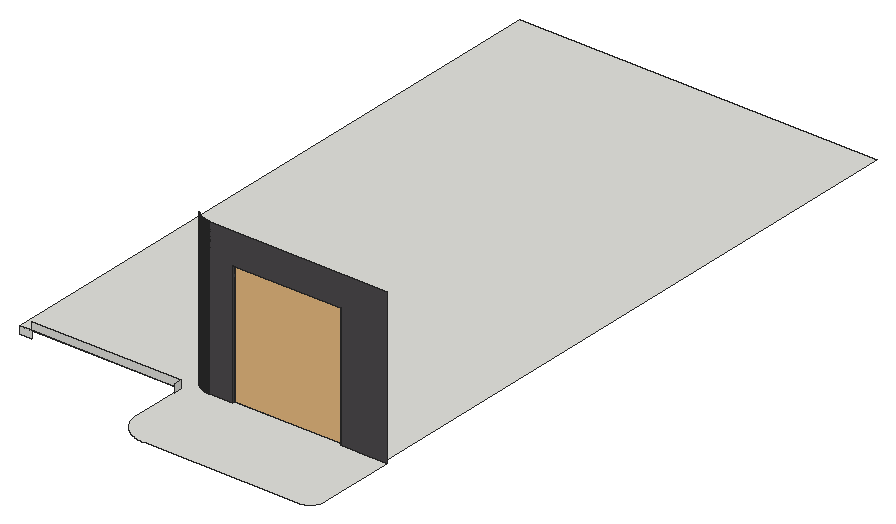
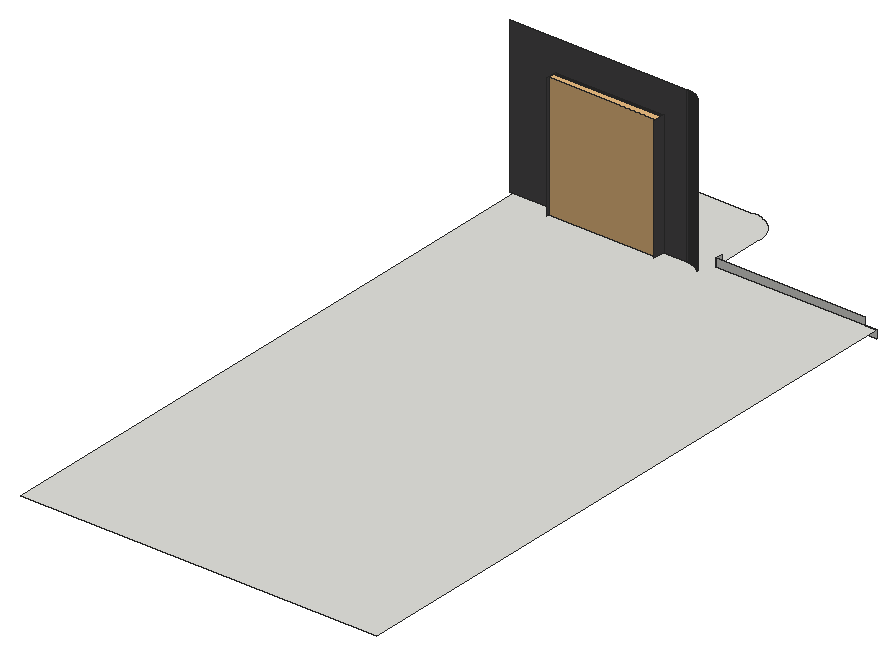
# SketchUp Ruby script. Lengths in inches.
U = 1.inch
M = Sketchup.active_model
def pt(a) = Geom::Point3d.new(a.map { |v| v * U })
def face(e, loops, mat)
  f = e.add_face(loops[0].map { |a| pt(a) })
  loops[1..].each { |l| e.add_face(l.map { |a| pt(a) }).erase! }
  f.material = f.back_material = mat if mat
  f
end
# faces: each face lists its corners as indices into pts; further lists are holes
def faces(e, pts, list, mat = nil) = list.each { |f| face(e, (f[0].is_a?(Array) ? f : [f]).map { |l| l.map { |i| pts[i] } }, mat) }
# xy, xz, yz: faces in a plane at the given z, y or x. An outline is a flat list of corners, or four numbers for a rectangle; further outlines are holes
def ring(l) = l.size == 4 ? [[l[0], l[1]], [l[2], l[1]], [l[2], l[3]], [l[0], l[3]]] : l.each_slice(2).to_a
def flat(e, list, mat, &to3) = list.each { |f| face(e, (f[0].is_a?(Array) ? f : [f]).map { |l| ring(l).map { |u, v| to3.(u, v) } }, mat) }
def xy(e, z, list, mat = nil) = flat(e, list, mat) { |x, y| [x, y, z] }
def xz(e, y, list, mat = nil) = flat(e, list, mat) { |x, z| [x, y, z] }
def yz(e, x, list, mat = nil) = flat(e, list, mat) { |y, z| [x, y, z] }
def lines(e, pts, list) = list.each { |a, b| e.add_line(pt(pts[a]), pt(pts[b])) }
# prism: a flat outline (further loops are holes) pulled along v
def prism(e, loops, v, mat = nil)
  f = face(e, loops, mat); d = Geom::Vector3d.new(v.map { |x| x * U })
  f.pushpull(f.normal.samedirection?(d) ? d.length : -d.length)
end
def box(e, o, s, mat = nil) = prism(e, [[o, [o[0] + s[0], o[1], o[2]], [o[0] + s[0], o[1] + s[1], o[2]], [o[0], o[1] + s[1], o[2]]]], [0, 0, s[2]], mat)
def at(x, y, z, deg = 0) = Geom::Transformation.translation(pt([x, y, z])) * Geom::Transformation.rotation(ORIGIN, Z_AXIS, deg.degrees)
def axes(o, x, y, z) = Geom::Transformation.new([*x, 0, *y, 0, *z, 0, *pt(o).to_a, 1])
def part(name) = M.definitions.add(name)
# library, detail: a bought-in or finely detailed component or shape, given as its bounding box
def library(name, o, s) = part(name).tap { |d| box(d.entities, o, s) }
def detail(e, o, s) = box(e.add_group.entities, o, s)
def put(e, d, t, mat = nil) = e.add_instance(d, t).tap { |i| i.material = mat if mat }
def group(e, t, mat = nil) = e.add_group.tap { |g| g.transformation = t; g.material = mat if mat }.entities
root = M.entities
M.materials.add("1423 AP 8230 BENTONITE").color = [77, 75, 77]
c1 = library("Untitled",[0,0,0],[96,5.09,80])
xy(root,119,[[159.84,137.5,159.76,137.51,159.6875,137.52,159.61,137.53,159.53,137.54,159.45,137.56,159.38,137.58,159.3,137.6,159.23,137.62,159.15,137.65,159.01,137.71,158.9375,137.74,158.87,137.77,158.59,137.93,158.53,137.98,158.47,138.02,158.41,138.07,158.29,138.18,158.23,138.23,158.18,138.29,158.07,138.41,158.02,138.47,157.98,138.53,157.93,138.59,157.77,138.87,157.74,138.9375,157.71,139.01,157.65,139.15,157.62,139.23,157.6,139.3,157.58,139.38,157.56,139.45,157.54,139.53,157.53,139.61,157.52,139.6875,157.51,139.76,157.5,139.84,157.5,140.16,157.51,140.24,157.52,140.3125,157.53,140.39,157.54,140.47,157.56,140.55,157.58,140.62,157.6,140.7,157.62,140.77,157.65,140.85,157.71,140.99,157.74,141.0625,157.77,141.13,157.93,141.41,157.98,141.47,158.02,141.53,158.07,141.59,158.18,141.71,158.23,141.77,158.29,141.82,158.41,141.93,158.47,141.98,158.53,142.02,158.59,142.07,158.87,142.23,158.9375,142.26,159.01,142.29,159.15,142.35,159.23,142.38,159.3,142.4,159.38,142.42,159.45,142.44,159.53,142.46,159.61,142.47,159.6875,142.48,159.76,142.49,159.84,142.5,160.16,142.5,160.24,142.49,160.3125,142.48,160.39,142.47,160.47,142.46,160.55,142.44,160.62,142.42,160.7,142.4,160.77,142.38,160.85,142.35,160.99,142.29,161.0625,142.26,161.13,142.23,161.41,142.07,161.47,142.02,161.53,141.98,161.59,141.93,161.71,141.82,161.77,141.77,161.82,141.71,161.93,141.59,161.98,141.53,162.02,141.47,162.07,141.41,162.23,141.13,162.26,141.0625,162.29,140.99,162.35,140.85,162.38,140.77,162.4,140.7,162.42,140.62,162.44,140.55,162.46,140.47,162.47,140.39,162.48,140.3125,162.49,140.24,162.5,140.16,162.5,139.84,162.49,139.76,162.48,139.6875,162.47,139.61,162.46,139.53,162.44,139.45,162.42,139.38,162.4,139.3,162.38,139.23,162.35,139.15,162.29,139.01,162.26,138.9375,162.23,138.87,162.07,138.59,162.02,138.53,161.98,138.47,161.93,138.41,161.82,138.29,161.77,138.23,161.71,138.18,161.59,138.07,161.53,138.02,161.47,137.98,161.41,137.93,161.13,137.77,161.0625,137.74,160.99,137.71,160.85,137.65,160.77,137.62,160.7,137.6,160.62,137.58,160.55,137.56,160.47,137.54,160.39,137.53,160.3125,137.52,160.24,137.51,160.16,137.5],[263.84,137.5,263.76,137.51,263.6875,137.52,263.61,137.53,263.53,137.54,263.45,137.56,263.38,137.58,263.3,137.6,263.23,137.62,263.15,137.65,262.94,137.74,262.86,137.77,262.8,137.81,262.59,137.93,262.53,137.98,262.47,138.02,262.41,138.07,262.29,138.18,262.23,138.23,262.18,138.29,262.07,138.41,262.02,138.47,261.98,138.53,261.93,138.59,261.77,138.87,261.74,138.9375,261.71,139.01,261.65,139.15,261.62,139.23,261.6,139.3,261.58,139.38,261.56,139.45,261.54,139.53,261.53,139.61,261.52,139.6875,261.51,139.76,261.5,139.84,261.5,140.16,261.51,140.24,261.52,140.3125,261.53,140.39,261.54,140.47,261.56,140.55,261.58,140.62,261.6,140.7,261.62,140.77,261.65,140.85,261.71,140.99,261.74,141.0625,261.77,141.13,261.93,141.41,261.98,141.47,262.02,141.53,262.07,141.59,262.18,141.71,262.23,141.77,262.29,141.82,262.41,141.93,262.47,141.98,262.53,142.02,262.59,142.07,262.8,142.19,262.86,142.23,262.94,142.26,263.15,142.35,263.23,142.38,263.3,142.4,263.38,142.42,263.45,142.44,263.53,142.46,263.61,142.47,263.6875,142.48,263.76,142.49,263.84,142.5,264.16,142.5,264.24,142.49,264.3125,142.48,264.39,142.47,264.47,142.46,264.55,142.44,264.62,142.42,264.7,142.4,264.77,142.38,264.85,142.35,264.99,142.29,265.0625,142.26,265.13,142.23,265.41,142.07,265.47,142.02,265.53,141.98,265.59,141.93,265.71,141.82,265.77,141.77,265.82,141.71,265.93,141.59,265.98,141.53,266.02,141.47,266.07,141.41,266.23,141.13,266.26,141.0625,266.29,140.99,266.35,140.85,266.38,140.77,266.4,140.7,266.42,140.62,266.44,140.55,266.46,140.47,266.47,140.39,266.48,140.3125,266.49,140.24,266.49,140.16,266.5,140.08,266.5,139.92,266.49,139.84,266.49,139.76,266.48,139.6875,266.47,139.61,266.46,139.53,266.44,139.45,266.42,139.38,266.4,139.3,266.38,139.23,266.35,139.15,266.29,139.01,266.26,138.9375,266.23,138.87,266.07,138.59,266.02,138.53,265.98,138.47,265.93,138.41,265.82,138.29,265.77,138.23,265.71,138.18,265.59,138.07,265.53,138.02,265.47,137.98,265.41,137.93,265.13,137.77,265.0625,137.74,264.99,137.71,264.85,137.65,264.77,137.62,264.7,137.6,264.62,137.58,264.55,137.56,264.47,137.54,264.39,137.53,264.3125,137.52,264.24,137.51,264.16,137.5],[159.84,169.5,159.76,169.51,159.6875,169.52,159.61,169.53,159.53,169.54,159.45,169.56,159.38,169.58,159.3,169.6,159.23,169.62,159.15,169.65,159.01,169.71,158.9375,169.74,158.87,169.77,158.59,169.93,158.53,169.98,158.47,170.02,158.41,170.07,158.29,170.18,158.23,170.23,158.18,170.29,158.07,170.41,158.02,170.47,157.98,170.53,157.93,170.59,157.77,170.87,157.74,170.9375,157.71,171.01,157.65,171.15,157.62,171.23,157.6,171.3,157.58,171.38,157.56,171.45,157.54,171.53,157.53,171.61,157.52,171.6875,157.51,171.76,157.5,171.84,157.5,172.16,157.51,172.24,157.52,172.3125,157.53,172.39,157.54,172.47,157.56,172.55,157.58,172.62,157.6,172.7,157.62,172.77,157.65,172.85,157.71,172.99,157.74,173.0625,157.77,173.13,157.93,173.41,157.98,173.47,158.02,173.53,158.07,173.59,158.18,173.71,158.23,173.77,158.29,173.82,158.41,173.93,158.47,173.98,158.53,174.02,158.59,174.07,158.87,174.23,158.9375,174.26,159.01,174.29,159.15,174.35,159.23,174.38,159.3,174.4,159.38,174.42,159.45,174.44,159.53,174.46,159.61,174.47,159.6875,174.48,159.76,174.49,159.84,174.5,160.16,174.5,160.24,174.49,160.3125,174.48,160.39,174.47,160.47,174.46,160.55,174.44,160.62,174.42,160.7,174.4,160.77,174.38,160.85,174.35,160.99,174.29,161.0625,174.26,161.13,174.23,161.41,174.07,161.47,174.02,161.53,173.98,161.59,173.93,161.71,173.82,161.77,173.77,161.82,173.71,161.93,173.59,161.98,173.53,162.02,173.47,162.07,173.41,162.23,173.13,162.26,173.0625,162.29,172.99,162.35,172.85,162.38,172.77,162.4,172.7,162.42,172.62,162.44,172.55,162.46,172.47,162.47,172.39,162.48,172.3125,162.49,172.24,162.5,172.16,162.5,171.84,162.49,171.76,162.48,171.6875,162.47,171.61,162.46,171.53,162.44,171.45,162.42,171.38,162.4,171.3,162.38,171.23,162.35,171.15,162.29,171.01,162.26,170.9375,162.23,170.87,162.07,170.59,162.02,170.53,161.98,170.47,161.93,170.41,161.82,170.29,161.77,170.23,161.71,170.18,161.59,170.07,161.53,170.02,161.47,169.98,161.41,169.93,161.13,169.77,161.0625,169.74,160.99,169.71,160.85,169.65,160.77,169.62,160.7,169.6,160.62,169.58,160.55,169.56,160.47,169.54,160.39,169.53,160.3125,169.52,160.24,169.51,160.16,169.5],[263.84,169.5,263.76,169.51,263.6875,169.52,263.61,169.53,263.53,169.54,263.45,169.56,263.38,169.58,263.3,169.6,263.23,169.62,263.15,169.65,262.94,169.74,262.86,169.77,262.8,169.81,262.59,169.93,262.53,169.98,262.47,170.02,262.41,170.07,262.29,170.18,262.23,170.23,262.18,170.29,262.07,170.41,262.02,170.47,261.98,170.53,261.93,170.59,261.77,170.87,261.74,170.9375,261.71,171.01,261.65,171.15,261.62,171.23,261.6,171.3,261.58,171.38,261.56,171.45,261.54,171.53,261.53,171.61,261.52,171.6875,261.51,171.76,261.5,171.84,261.5,172.16,261.51,172.24,261.52,172.3125,261.53,172.39,261.54,172.47,261.56,172.55,261.58,172.62,261.6,172.7,261.62,172.77,261.65,172.85,261.71,172.99,261.74,173.0625,261.77,173.13,261.93,173.41,261.98,173.47,262.02,173.53,262.07,173.59,262.18,173.71,262.23,173.77,262.29,173.82,262.41,173.93,262.47,173.98,262.53,174.02,262.59,174.07,262.8,174.19,262.86,174.23,262.94,174.26,263.15,174.35,263.23,174.38,263.3,174.4,263.38,174.42,263.45,174.44,263.53,174.46,263.61,174.47,263.6875,174.48,263.76,174.49,263.84,174.5,264.16,174.5,264.24,174.49,264.3125,174.48,264.39,174.47,264.47,174.46,264.55,174.44,264.62,174.42,264.7,174.4,264.77,174.38,264.85,174.35,264.99,174.29,265.0625,174.26,265.13,174.23,265.41,174.07,265.47,174.02,265.53,173.98,265.59,173.93,265.71,173.82,265.77,173.77,265.82,173.71,265.93,173.59,265.98,173.53,266.02,173.47,266.07,173.41,266.23,173.13,266.26,173.0625,266.29,172.99,266.35,172.85,266.38,172.77,266.4,172.7,266.42,172.62,266.44,172.55,266.46,172.47,266.47,172.39,266.48,172.3125,266.49,172.24,266.49,172.16,266.5,172.08,266.5,171.92,266.49,171.84,266.49,171.76,266.48,171.6875,266.47,171.61,266.46,171.53,266.44,171.45,266.42,171.38,266.4,171.3,266.38,171.23,266.35,171.15,266.29,171.01,266.26,170.9375,266.23,170.87,266.07,170.59,266.02,170.53,265.98,170.47,265.93,170.41,265.82,170.29,265.77,170.23,265.71,170.18,265.59,170.07,265.53,170.02,265.47,169.98,265.41,169.93,265.13,169.77,265.0625,169.74,264.99,169.71,264.85,169.65,264.77,169.62,264.7,169.6,264.62,169.58,264.55,169.56,264.47,169.54,264.39,169.53,264.3125,169.52,264.24,169.51,264.16,169.5]])
xy(root,126,[[157.6875,120,278.24,120,278.47,120.01,278.71,120.02,278.94,120.04,279.18,120.06,279.41,120.08,279.64,120.11,279.88,120.15,280.11,120.1875,280.34,120.23,280.8,120.33,281.26,120.45,281.48,120.52,281.71,120.59,281.93,120.66,282.15,120.74,282.375,120.83,282.59,120.91,282.81,121.01,283.02,121.1,283.24,121.2,283.66,121.42,283.86,121.53,284.07,121.65,284.47,121.89,284.67,122.02,284.86,122.16,285.05,122.29,285.24,122.43,285.43,122.58,285.61,122.72,285.97,123.03,286.15,123.1875,286.32,123.35,286.49,123.51,286.65,123.68,286.8125,123.85,286.97,124.03,287.28,124.39,287.42,124.57,287.57,124.76,287.71,124.95,287.84,125.14,287.98,125.33,288.11,125.53,288.35,125.93,288.47,126.14,288.58,126.34,288.8,126.76,288.9,126.98,288.99,127.19,289.09,127.41,289.17,127.625,289.26,127.85,289.34,128.07,289.41,128.29,289.48,128.52,289.55,128.74,289.67,129.2,289.77,129.66,289.8125,129.89,289.85,130.12,289.89,130.36,289.92,130.59,289.94,130.82,289.96,131.06,289.98,131.29,289.99,131.53,290,131.76,290,192,287,192,287,672,9,672,9,186,134,186,134,143.6875,134.01,143.37,134.02,143.06,134.03,142.74,134.07,142.12,134.1,141.8,134.13,141.49,134.25,140.56,134.3,140.25,134.4,139.625,134.46,139.32,134.52,139.01,134.59,138.7,134.66,138.4,134.74,138.09,134.9,137.49,134.99,137.18,135.17,136.58,135.27,136.29,135.48,135.69,135.59,135.4,136.07,134.24,136.2,133.95,136.48,133.39,136.62,133.1,136.76,132.83,137.06,132.27,137.22,132,137.375,131.73,137.54,131.46,137.7,131.19,138.04,130.67,138.58,129.89,139.15,129.14,139.35,128.9,139.55,128.65,139.75,128.41,139.96,128.18,140.16,127.94,140.59,127.48,140.81,127.25,141.25,126.81,141.48,126.59,141.94,126.16,142.18,125.96,142.41,125.75,142.65,125.55,142.9,125.35,143.14,125.15,143.89,124.58,144.67,124.04,145.19,123.7,145.46,123.54,145.73,123.375,146,123.22,146.27,123.06,146.83,122.76,147.1,122.62,147.39,122.48,147.95,122.2,148.24,122.07,149.4,121.59,149.69,121.48,150.29,121.27,150.58,121.17,151.18,120.99,151.49,120.9,152.09,120.74,152.4,120.66,152.7,120.59,153.01,120.52,153.32,120.46,153.625,120.4,154.25,120.3,154.56,120.25,155.49,120.13,155.8,120.1,156.12,120.07,156.74,120.03,157.06,120.02,157.37,120.01]])
xz(root,186,[[9,120,18,126],[18,126,134,132]])
xz(root,192,[[151.78,126,152,246],[152,126,170,126,170,222,254,222,254,126,290,126,290,246,152,246]],"1423 AP 8230 BENTONITE")
xz(root,192.01,[[151.35,126,151.57,246]],"1423 AP 8230 BENTONITE")
yz(root,134,[[180,126,186,132]])
yz(root,170,[[192,126,201,222]],"1423 AP 8230 BENTONITE")
yz(root,254,[[192,126,201,222]],"1423 AP 8230 BENTONITE")
p = [[150.7,192.05,246],[150.48,192.0625,246],[150.48,192.0625,126],[150.7,192.05,126],[150.91,192.03,246],[150.91,192.03,126],
  [151.13,192.02,246],[151.13,192.02,126],[151.35,192.01,246],[151.35,192.01,126],[151.78,192,246],[151.57,192.01,246],
  [151.57,192.01,126],[151.78,192,126],[149.83,192.13,246],[149.61,192.16,246],[149.61,192.16,126],[149.83,192.13,126],
  [150.05,192.11,246],[150.05,192.11,126],[150.26,192.08,246],[150.26,192.08,126],[149.18,192.22,246],[148.97,192.26,246],
  [148.97,192.26,126],[149.18,192.22,126],[149.4,192.1875,246],[149.4,192.1875,126],[148.54,192.34,246],[148.33,192.38,246],
  [148.33,192.38,126],[148.54,192.34,126],[148.76,192.29,246],[148.76,192.29,126],[148.12,192.42,246],[147.9,192.47,246],
  [147.9,192.47,126],[148.12,192.42,126],[147.69,192.52,246],[147.48,192.58,246],[147.48,192.58,126],[147.69,192.52,126],
  [147.27,192.63,246],[147.0625,192.69,246],[147.0625,192.69,126],[147.27,192.63,126],[146.85,192.75,246],[146.85,192.75,126],
  [146.64,192.82,246],[146.4375,192.88,246],[146.4375,192.88,126],[146.64,192.82,126],[146.23,192.95,246],[146.03,193.02,246],
  [146.03,193.02,126],[146.23,192.95,126],[145.82,193.09,246],[145.82,193.09,126],[145.62,193.17,246],[145.62,193.17,126],
  [145.41,193.25,246],[145.21,193.33,246],[145.21,193.33,126],[145.41,193.25,126],[145.01,193.41,246],[145.01,193.41,126],
  [144.8125,193.5,246],[144.8125,193.5,126],[144.61,193.59,246],[144.61,193.59,126],[144.41,193.68,246],[144.41,193.68,126],
  [144.22,193.77,246],[144.22,193.77,126],[144.02,193.86,246],[144.02,193.86,126],[143.83,193.96,246],[143.83,193.96,126],
  [143.63,194.0625,246],[143.63,194.0625,126],[143.44,194.16,246],[143.44,194.16,126],[143.25,194.27,246],[143.25,194.27,126],
  [143.0625,194.375,246],[143.0625,194.375,126],[142.875,194.48,246],[142.875,194.48,126],[142.6875,194.6,246],[142.6875,194.6,126],
  [142.5,194.71,246],[142.5,194.71,126],[142.32,194.83,246],[142.32,194.83,126],[142.14,194.94,246],[142.14,194.94,126],
  [141.95,195.0625,246],[141.95,195.0625,126],[141.77,195.1875,246],[141.77,195.1875,126],[141.6,195.3125,246],[141.6,195.3125,126],
  [141.42,195.4375,246],[141.42,195.4375,126],[141.24,195.57,246],[141.24,195.57,126],[141.07,195.7,246],[141.07,195.7,126],
  [140.9,195.83,246],[140.9,195.83,126],[140.73,195.97,246],[140.73,195.97,126],[140.56,196.1,246],[140.56,196.1,126],
  [140.39,196.24,246],[140.39,196.24,126],[140.23,196.38,246],[140.23,196.38,126],[140.0625,196.53,246],[140.0625,196.53,126],
  [139.9,196.67,246],[139.9,196.67,126],[139.74,196.82,246],[139.74,196.82,126],[139.58,196.97,246],[139.58,196.97,126],
  [139.43,197.12,246],[139.43,197.12,126],[139.27,197.27,246],[139.27,197.27,126],[151.97,192,120],[151.97,192,126],
  [134,209.97,120],[134,180,120]]
faces(root,p,[[0,1,2,3],[4,0,3,5],[6,4,5,7],[8,6,7,9],[10,11,12,13],[14,15,16,17],[18,14,17,19],[20,18,19,21],
  [1,20,21,2],[22,23,24,25],[26,22,25,27],[15,26,27,16],[28,29,30,31],[32,28,31,33],[23,32,33,24],[34,35,36,37],
  [29,34,37,30],[38,39,40,41],[35,38,41,36],[42,43,44,45],[39,42,45,40],[43,46,47,44],[48,49,50,51],[46,48,51,47],
  [52,53,54,55],[49,52,55,50],[53,56,57,54],[56,58,59,57],[60,61,62,63],[58,60,63,59],[61,64,65,62],[64,66,67,65],
  [66,68,69,67],[68,70,71,69],[70,72,73,71],[72,74,75,73],[74,76,77,75],[76,78,79,77],[78,80,81,79],[80,82,83,81],
  [82,84,85,83],[84,86,87,85],[86,88,89,87],[88,90,91,89],[90,92,93,91],[92,94,95,93],[94,96,97,95],[96,98,99,97],
  [98,100,101,99],[100,102,103,101],[102,104,105,103],[104,106,107,105],[106,108,109,107],[108,110,111,109],[110,112,113,111],[112,114,115,113],
  [114,116,117,115],[116,118,119,117],[118,120,121,119],[120,122,123,121],[122,124,125,123],[124,126,127,125],[126,128,129,127]],"1423 AP 8230 BENTONITE")
lines(root,p,[[130,131],[132,133]])
put(root,c1,axes([170,194,126],[0.875,0,0],[0,1,0],[0,0,1.2]),"1423 AP 8230 BENTONITE")
